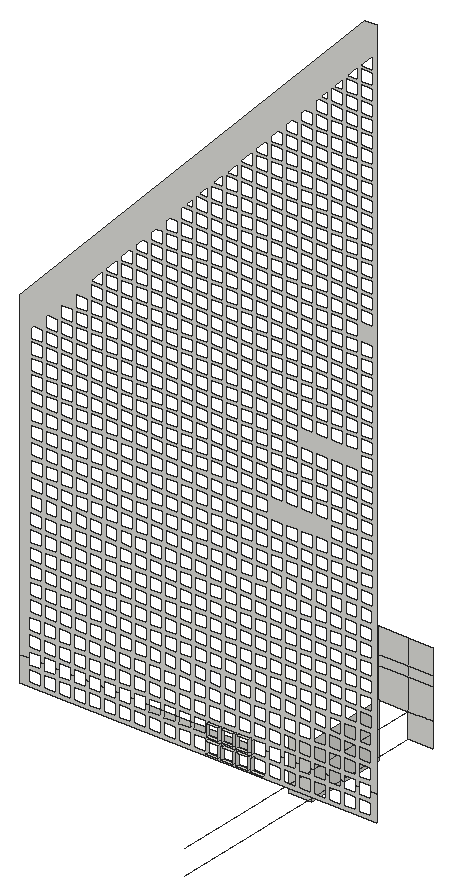
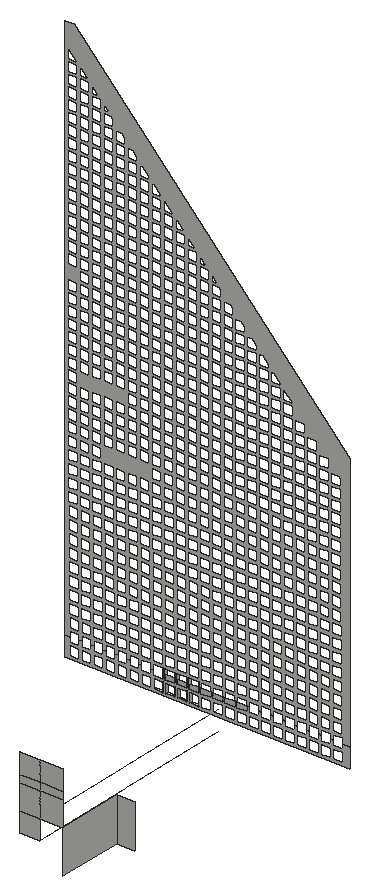
# SketchUp Ruby script. Lengths in inches.
U = 1.inch
M = Sketchup.active_model
def pt(a) = Geom::Point3d.new(a.map { |v| v * U })
def face(e, loops, mat)
  f = e.add_face(loops[0].map { |a| pt(a) })
  loops[1..].each { |l| e.add_face(l.map { |a| pt(a) }).erase! }
  f.material = f.back_material = mat if mat
  f
end
# faces: each face lists its corners as indices into pts; further lists are holes
def faces(e, pts, list, mat = nil) = list.each { |f| face(e, (f[0].is_a?(Array) ? f : [f]).map { |l| l.map { |i| pts[i] } }, mat) }
# xy, xz, yz: faces in a plane at the given z, y or x. An outline is a flat list of corners, or four numbers for a rectangle; further outlines are holes
def ring(l) = l.size == 4 ? [[l[0], l[1]], [l[2], l[1]], [l[2], l[3]], [l[0], l[3]]] : l.each_slice(2).to_a
def flat(e, list, mat, &to3) = list.each { |f| face(e, (f[0].is_a?(Array) ? f : [f]).map { |l| ring(l).map { |u, v| to3.(u, v) } }, mat) }
def xy(e, z, list, mat = nil) = flat(e, list, mat) { |x, y| [x, y, z] }
def xz(e, y, list, mat = nil) = flat(e, list, mat) { |x, z| [x, y, z] }
def yz(e, x, list, mat = nil) = flat(e, list, mat) { |y, z| [x, y, z] }
def lines(e, pts, list) = list.each { |a, b| e.add_line(pt(pts[a]), pt(pts[b])) }
# prism: a flat outline (further loops are holes) pulled along v
def prism(e, loops, v, mat = nil)
  f = face(e, loops, mat); d = Geom::Vector3d.new(v.map { |x| x * U })
  f.pushpull(f.normal.samedirection?(d) ? d.length : -d.length)
end
def box(e, o, s, mat = nil) = prism(e, [[o, [o[0] + s[0], o[1], o[2]], [o[0] + s[0], o[1] + s[1], o[2]], [o[0], o[1] + s[1], o[2]]]], [0, 0, s[2]], mat)
def at(x, y, z, deg = 0) = Geom::Transformation.translation(pt([x, y, z])) * Geom::Transformation.rotation(ORIGIN, Z_AXIS, deg.degrees)
def axes(o, x, y, z) = Geom::Transformation.new([*x, 0, *y, 0, *z, 0, *pt(o).to_a, 1])
def part(name) = M.definitions.add(name)
# library, detail: a bought-in or finely detailed component or shape, given as its bounding box
def library(name, o, s) = part(name).tap { |d| box(d.entities, o, s) }
def detail(e, o, s) = box(e.add_group.entities, o, s)
def put(e, d, t, mat = nil) = e.add_instance(d, t).tap { |i| i.material = mat if mat }
def group(e, t, mat = nil) = e.add_group.tap { |g| g.transformation = t; g.material = mat if mat }.entities
root = M.entities
xy(root,259.68,[[986.41,2332.13,988.72,2332.76],[989.32,2332.13,991.63,2332.76],[992.23,2332.13,994.55,2332.76],[995.15,2332.13,997.46,2332.76]])
xy(root,262,[[986.41,2332.13,988.72,2332.76],[989.32,2332.13,991.63,2332.76],[992.23,2332.13,994.55,2332.76]])
xy(root,262.73,[[986.4375,2332.13,988.75,2332.76],[989.35,2332.13,991.66,2332.76],[992.26,2332.13,994.58,2332.76]])
xy(root,265.04,[[986.4375,2332.13,988.75,2332.76],[989.35,2332.13,991.66,2332.76],[992.26,2332.13,994.58,2332.76]])
xz(root,2332.76,[[[949.71,258.95,949.71,263.89,951.49,263.89,951.49,262.73,953.81,262.73,953.81,263.89,954.41,263.89,954.41,262.73,956.72,262.73,956.72,263.89,957.32,263.89,957.32,262.73,959.63,262.73,959.63,263.89,960.23,263.89,960.23,262.73,962.54,262.73,962.54,263.89,963.14,263.89,963.14,262.73,965.46,262.73,965.46,263.89,966.06,263.89,966.06,262.73,968.37,262.73,968.37,263.89,968.97,263.89,968.97,262.73,971.28,262.73,971.28,263.89,971.88,263.89,971.88,262.73,974.19,262.73,974.19,263.89,974.79,263.89,974.79,262.73,977.1,262.73,977.1,263.89,977.7,263.89,977.7,262.73,980.02,262.73,980.02,263.89,980.62,263.89,980.62,262.73,982.93,262.73,982.93,263.89,983.53,263.89,983.53,262.73,985.84,262.73,985.84,263.89,986.4375,263.89,986.4375,262.73,988.75,262.73,988.75,263.89,989.35,263.89,989.35,262.73,991.66,262.73,991.66,263.89,992.26,263.89,992.26,262.73,994.58,262.73,994.58,263.89,995.18,263.89,995.18,262.73,997.49,262.73,997.49,263.89,998.09,263.89,998.09,262.73,1000.4,262.73,1000.4,263.89,1001,263.89,1001,262.73,1003.3125,262.73,1003.3125,263.89,1003.91,263.89,1003.91,262.73,1006.22,262.73,1006.22,263.89,1006.82,263.89,1006.82,262.73,1009.14,262.73,1009.14,263.89,1009.74,263.89,1009.74,262.73,1012.05,262.73,1012.05,263.89,1012.65,263.89,1012.65,262.73,1014.96,262.73,1014.96,263.89,1015.56,263.89,1015.56,262.73,1017.87,262.73,1017.87,263.89,1019.02,263.89,1019.02,258.95],[1015.53,259.68,1017.84,262],[1012.62,259.68,1014.93,262],[1009.71,259.68,1012.02,262],[1006.79,259.68,1009.11,262],[1003.88,259.68,1006.2,262],[1000.97,259.68,1003.28,262],[998.06,259.68,1000.37,262],[995.15,259.68,997.46,262],[992.23,259.68,994.55,262],[989.32,259.68,991.63,262],[986.41,259.68,988.72,262],[983.5,259.68,985.8125,262],[980.59,259.68,982.9,262],[977.67,259.68,979.99,262],[974.76,259.68,977.07,262],[971.85,259.68,974.16,262],[968.9375,259.68,971.25,262],[966.03,259.68,968.34,262],[963.11,259.68,965.43,262],[960.2,259.68,962.51,262],[957.29,259.68,959.6,262],[954.38,259.68,956.69,262],[951.47,259.68,953.78,262]],[974.79,262.73,977.1,263.89],[977.7,262.73,980.02,263.89],[980.62,262.73,982.93,263.89],[983.53,262.73,985.84,263.89],
  [986.4375,262.73,988.75,263.89],[989.35,262.73,991.66,263.89],[992.26,262.73,994.58,263.89],[[949.71,263.89,949.71,326.5,1016.77,397.75,1019.02,397.75,1019.02,263.89,1017.87,263.89,1017.87,265.04,1015.56,265.04,1015.56,263.89,1014.96,263.89,1014.96,265.04,1012.65,265.04,1012.65,263.89,1012.05,263.89,1012.05,265.04,1009.74,265.04,1009.74,263.89,1009.14,263.89,1009.14,265.04,1006.82,265.04,1006.82,263.89,1006.22,263.89,1006.22,265.04,1003.91,265.04,1003.91,263.89,1003.3125,263.89,1003.3125,265.04,1001,265.04,1001,263.89,1000.4,263.89,1000.4,265.04,998.09,265.04,998.09,263.89,997.49,263.89,997.49,265.04,995.18,265.04,995.18,263.89,994.58,263.89,994.58,265.04,992.26,265.04,992.26,263.89,991.66,263.89,991.66,265.04,989.35,265.04,989.35,263.89,988.75,263.89,988.75,265.04,986.4375,265.04,986.4375,263.89,985.84,263.89,985.84,265.04,983.53,265.04,983.53,263.89,982.93,263.89,982.93,265.04,980.62,265.04,980.62,263.89,980.02,263.89,980.02,265.04,977.7,265.04,977.7,263.89,977.1,263.89,977.1,265.04,974.79,265.04,974.79,263.89,974.19,263.89,974.19,265.04,971.88,265.04,971.88,263.89,971.28,263.89,971.28,265.04,968.97,265.04,968.97,263.89,968.37,263.89,968.37,265.04,966.06,265.04,966.06,263.89,965.46,263.89,965.46,265.04,963.14,265.04,963.14,263.89,962.54,263.89,962.54,265.04,960.23,265.04,960.23,263.89,959.63,263.89,959.63,265.04,957.32,265.04,957.32,263.89,956.72,263.89,956.72,265.04,954.41,265.04,954.41,263.89,953.81,263.89,953.81,265.04,951.49,265.04,951.49,263.89],[1004.32,370.27,1006.66,372.59],[1015.99,386.84,1018.31,389.15],[1015.99,384.09,1018.31,386.4],[1013.08,384.09,1015.4,386.4],[1013.06,381.34,1015.37,383.65],[1015.99,381.34,1018.31,383.65],[1015.99,378.59,1018.31,380.9],[1013.06,378.59,1015.37,380.9],[1010.15,375.84,1012.46,378.15],[1013.08,375.84,1015.4,378.15],[1015.99,375.84,1018.31,378.15],[1015.99,373.09,1018.31,375.4],[1013.06,373.09,1015.37,375.4],[1010.17,373.09,1012.48,375.4],[1007.23,373.09,1009.55,375.4],[1013.06,370.27,1015.37,372.59],[1015.99,370.27,1018.31,372.59],[1007.26,370.27,1009.57,372.59],[1001.43,370.27,1003.75,372.59],[998.52,367.46,1000.83,369.77],[1001.43,367.46,1003.75,369.77],[1004.35,367.46,1006.66,369.77],[1007.26,367.46,1009.57,369.77],[1010.17,367.46,1012.48,369.77],[1013.08,367.46,1015.4,369.77],[1015.99,367.46,1018.31,369.77],[1015.99,364.65,1018.31,366.96],[1013.08,364.65,1015.4,366.96],[1010.17,364.65,1012.48,366.96],[1007.26,364.65,1009.57,366.96],[1004.35,364.65,1006.66,366.96],[1001.43,364.65,1003.75,366.96],[998.52,364.65,1000.83,366.96],[995.61,364.65,997.92,366.96],[992.7,361.84,995.01,364.15],[995.61,361.84,997.92,364.15],[998.52,361.84,1000.83,364.15],[1001.43,361.84,1003.75,364.15],[1004.35,361.84,1006.66,364.15],[1007.26,361.84,1009.57,364.15],[1010.17,361.84,1012.48,364.15],[1013.08,361.84,1015.4,364.15],[1015.99,361.84,1018.31,364.15],[1015.99,359.02,1018.31,361.34],[1013.08,359.02,1015.4,361.34],[1010.17,359.02,1012.48,361.34],[1007.26,359.02,1009.57,361.34],[1004.35,359.02,1006.66,361.34],[1001.43,359.02,1003.75,361.34],[998.52,359.02,1000.83,361.34],[995.61,359.02,997.92,361.34],[992.7,359.02,995.01,361.34],[989.79,359.02,992.1,361.34],[986.875,356.21,989.1875,358.52],[989.79,356.21,992.1,358.52],[992.7,356.21,995.01,358.52],[995.61,356.21,997.92,358.52],[998.52,356.21,1000.83,358.52],[1001.43,356.21,1003.75,358.52],[1004.35,356.21,1006.66,358.52],[1007.26,356.21,1009.57,358.52],[1010.17,356.21,1012.48,358.52],[1013.08,356.21,1015.4,358.52],[1015.99,356.21,1018.31,358.52],[983.96,350.59,986.27,352.9],[986.875,353.4,989.1875,355.71],[986.875,350.59,989.1875,352.9],[989.79,350.59,992.1,352.9],[989.79,353.4,992.1,355.71],[992.7,353.4,995.01,355.71],[992.7,350.59,995.01,352.9],[995.61,353.4,997.92,355.71],[995.61,350.59,997.92,352.9],[998.52,353.4,1000.83,355.71],[998.52,350.59,1000.83,352.9],[1001.43,353.4,1003.75,355.71],[1001.43,350.59,1003.75,352.9],[1004.35,353.4,1006.66,355.71],[1004.35,350.59,1006.66,352.9],[1007.26,350.59,1009.57,352.9],[1007.26,353.4,1009.57,355.71],[1010.17,353.4,1012.48,355.71],[1013.08,353.4,1015.4,355.71],[1015.99,353.4,1018.31,355.71],[1015.99,350.59,1018.31,352.9],[1013.08,350.59,1015.4,352.9],[1010.17,350.59,1012.48,352.9],[1015.99,347.77,1018.31,350.09],[1013.08,347.77,1015.4,350.09],[1010.17,347.77,1012.48,350.09],[1007.26,347.77,1009.57,350.09],[1004.35,347.77,1006.66,350.09],[1001.43,347.77,1003.75,350.09],[998.52,347.77,1000.83,350.09],[995.61,347.77,997.92,350.09],[992.7,347.77,995.01,350.09],[989.79,347.77,992.1,350.09],[986.875,347.77,989.1875,350.09],[983.96,347.77,986.27,350.09],[981.05,347.77,983.36,350.09],[978.14,344.96,980.45,347.27],[981.05,344.96,983.36,347.27],[983.96,344.96,986.27,347.27],[986.875,344.96,989.1875,347.27],[989.79,344.96,992.1,347.27],[992.7,344.96,995.01,347.27],[995.61,344.96,997.92,347.27],[998.52,344.96,1000.83,347.27],[1001.43,344.96,1003.75,347.27],[1004.35,344.96,1006.66,347.27],[1007.26,344.96,1009.57,347.27],[1010.17,344.96,1012.48,347.27],[1013.08,344.96,1015.4,347.27],[1015.99,344.96,1018.31,347.27],[969.4,336.52,971.71,338.84],[972.3125,336.52,974.625,338.84],[975.23,336.52,977.54,338.84],[978.14,336.52,980.45,338.84],[981.05,336.52,983.36,338.84],[983.96,336.52,986.27,338.84],[986.875,336.52,989.1875,338.84],[989.79,336.52,992.1,338.84],[992.7,336.52,995.01,338.84],[995.61,336.52,997.92,338.84],[995.61,339.34,997.92,341.65],[992.7,339.34,995.01,341.65],[989.79,339.34,992.1,341.65],[986.875,339.34,989.1875,341.65],[983.96,339.34,986.27,341.65],[981.05,339.34,983.36,341.65],[978.14,339.34,980.45,341.65],[975.23,339.34,977.54,341.65],[972.3125,339.34,974.625,341.65],[975.23,342.15,977.54,344.46],[978.14,342.15,980.45,344.46],[981.05,342.15,983.36,344.46],[983.96,342.15,986.27,344.46],[986.875,342.15,989.1875,344.46],[989.79,342.15,992.1,344.46],[992.7,342.15,995.01,344.46],[995.61,342.15,997.92,344.46],[998.52,342.15,1000.83,344.46],[998.52,339.34,1000.83,341.65],[998.52,336.52,1000.83,338.84],[1001.43,336.52,1003.75,338.84],[1001.43,339.34,1003.75,341.65],[1001.43,342.15,1003.75,344.46],[1004.35,342.15,1006.66,344.46],[1004.35,339.34,1006.66,341.65],[1004.35,336.52,1006.66,338.84],[1007.26,336.52,1009.57,338.84],[1007.26,339.34,1009.57,341.65],[1007.26,342.15,1009.57,344.46],[1010.17,342.15,1012.48,344.46],[1010.17,339.34,1012.48,341.65],[1010.17,336.52,1012.48,338.84],[1013.08,336.52,1015.4,338.84],[1013.08,339.34,1015.4,341.65],[1013.08,342.15,1015.4,344.46],[1015.99,339.34,1018.31,341.65],[1015.99,336.52,1018.31,338.84],[1015.99,333.71,1018.31,336.02],[1013.08,333.71,1015.4,336.02],[1010.17,333.71,1012.48,336.02],[1007.26,333.71,1009.57,336.02],[1004.35,333.71,1006.66,336.02],[1001.43,333.71,1003.75,336.02],[998.52,333.71,1000.83,336.02],[995.61,333.71,997.92,336.02],[992.7,333.71,995.01,336.02],[989.79,333.71,992.1,336.02],[986.875,333.71,989.1875,336.02],[983.96,333.71,986.27,336.02],[981.05,333.71,983.36,336.02],[978.14,333.71,980.45,336.02],[975.23,333.71,977.54,336.02],[972.3125,333.71,974.625,336.02],[969.4,333.71,971.71,336.02],[966.49,333.71,968.8,336.02],[963.58,330.9,965.89,333.21],[966.49,330.9,968.8,333.21],[969.4,330.9,971.71,333.21],[972.3125,330.9,974.625,333.21],[975.23,330.9,977.54,333.21],[978.14,330.9,980.45,333.21],[981.05,330.9,983.36,333.21],[983.96,330.9,986.27,333.21],[986.875,330.9,989.1875,333.21],[989.79,330.9,992.1,333.21],[992.7,330.9,995.01,333.21],[995.61,330.9,997.92,333.21],[998.52,330.9,1000.83,333.21],[1001.43,330.9,1003.75,333.21],[1004.35,330.9,1006.66,333.21],[1007.26,330.9,1009.57,333.21],[1010.17,330.9,1012.48,333.21],[1013.08,330.9,1015.4,333.21],[1015.99,330.9,1018.31,333.21],[1015.99,328.09,1018.31,330.4],[1013.08,328.09,1015.4,330.4],[1010.17,328.09,1012.48,330.4],[1007.26,328.09,1009.57,330.4],[1004.35,328.09,1006.66,330.4],[1001.43,328.09,1003.75,330.4],[998.52,328.09,1000.83,330.4],[995.61,328.09,997.92,330.4],[992.7,328.09,995.01,330.4],[989.79,328.09,992.1,330.4],[986.875,328.09,989.1875,330.4],[983.96,328.09,986.27,330.4],[981.05,328.09,983.36,330.4],[978.14,328.09,980.45,330.4],[975.23,328.09,977.54,330.4],[972.3125,328.09,974.625,330.4],[969.4,328.09,971.71,330.4],[966.49,328.09,968.8,330.4],[963.58,328.09,965.89,330.4],[960.67,328.09,962.98,330.4],[957.75,325.27,960.07,327.59],[960.67,325.27,962.98,327.59],[963.58,325.27,965.89,327.59],[966.49,325.27,968.8,327.59],[969.4,325.27,971.71,327.59],[972.3125,325.27,974.625,327.59],[975.23,325.27,977.54,327.59],[978.14,325.27,980.45,327.59],[981.05,325.27,983.36,327.59],[983.96,325.27,986.27,327.59],[986.875,325.27,989.1875,327.59],[989.79,325.27,992.1,327.59],[992.7,325.27,995.01,327.59],[995.61,325.27,997.92,327.59],[998.52,325.27,1000.83,327.59],[1001.43,325.27,1003.75,327.59],[1004.35,325.27,1006.66,327.59],[1007.26,325.27,1009.57,327.59],[1010.17,325.27,1012.48,327.59],[1013.08,325.27,1015.4,327.59],[1015.99,325.27,1018.31,327.59],[1015.99,322.46,1018.31,324.77],[1013.08,322.46,1015.4,324.77],[1010.17,322.46,1012.48,324.77],[1007.26,322.46,1009.57,324.77],[1004.35,322.46,1006.66,324.77],[1001.43,322.46,1003.75,324.77],[998.52,322.46,1000.83,324.77],[995.61,322.46,997.92,324.77],[992.7,322.46,995.01,324.77],[989.79,322.46,992.1,324.77],[986.875,322.46,989.1875,324.77],[983.96,322.46,986.27,324.77],[981.05,322.46,983.36,324.77],[978.14,322.46,980.45,324.77],[978.14,319.65,980.45,321.96],[981.05,319.65,983.36,321.96],[983.96,319.65,986.27,321.96],[986.875,319.65,989.1875,321.96],[989.79,319.65,992.1,321.96],[992.7,319.65,995.01,321.96],[995.61,319.65,997.92,321.96],[998.52,319.65,1000.83,321.96],[1001.43,319.65,1003.75,321.96],[1015.99,319.65,1018.31,321.96],[1015.99,316.84,1018.31,319.15],[1013.08,316.84,1015.4,319.15],[1010.17,316.84,1012.48,319.15],[1007.26,316.84,1009.57,319.15],[1004.35,316.84,1006.66,319.15],[1001.43,316.84,1003.75,319.15],[998.52,316.84,1000.83,319.15],[995.61,316.84,997.92,319.15],[992.7,316.84,995.01,319.15],[989.79,316.84,992.1,319.15],[986.875,316.84,989.1875,319.15],[983.96,316.84,986.27,319.15],[981.05,316.84,983.36,319.15],[978.14,316.84,980.45,319.15],[978.14,314.02,980.45,316.34],[981.05,314.02,983.36,316.34],[983.96,314.02,986.27,316.34],[986.875,314.02,989.1875,316.34],[989.79,314.02,992.1,316.34],[992.7,314.02,995.01,316.34],[995.61,314.02,997.92,316.34],[998.52,314.02,1000.83,316.34],[1001.43,314.02,1003.75,316.34],[1004.35,314.02,1006.66,316.34],[1007.26,314.02,1009.57,316.34],[1010.17,314.02,1012.48,316.34],[1013.08,314.02,1015.4,316.34],[1015.99,314.02,1018.31,316.34],[957.75,322.46,960.07,324.77],[960.67,322.46,962.98,324.77],[963.58,322.46,965.89,324.77],[966.49,322.46,968.8,324.77],[969.4,322.46,971.71,324.77],[972.3125,322.46,974.625,324.77],[975.23,322.46,977.54,324.77],[975.23,319.65,977.54,321.96],[975.23,316.84,977.54,319.15],[975.23,314.02,977.54,316.34],[972.3125,314.02,974.625,316.34],[972.3125,316.84,974.625,319.15],[972.3125,319.65,974.625,321.96],[969.4,319.65,971.71,321.96],[966.49,319.65,968.8,321.96],[963.58,319.65,965.89,321.96],[960.67,319.65,962.98,321.96],[957.75,319.65,960.07,321.96],[954.84,319.65,957.15,321.96],[951.93,316.84,954.24,319.15],[954.84,316.84,957.15,319.15],[957.75,316.84,960.07,319.15],[960.67,316.84,962.98,319.15],[963.58,316.84,965.89,319.15],[966.49,316.84,968.8,319.15],[969.4,316.84,971.71,319.15],[969.4,314.02,971.71,316.34],[966.49,314.02,968.8,316.34],[963.58,314.02,965.89,316.34],[960.67,314.02,962.98,316.34],[957.75,314.02,960.07,316.34],[954.84,314.02,957.15,316.34],[951.93,314.02,954.24,316.34],[951.93,311.21,954.24,313.52],[954.84,311.21,957.15,313.52],[957.75,311.21,960.07,313.52],[960.67,311.21,962.98,313.52],[963.58,311.21,965.89,313.52],[966.49,311.21,968.8,313.52],[969.4,311.21,971.71,313.52],[972.3125,311.21,974.625,313.52],[975.23,311.21,977.54,313.52],[978.14,311.21,980.45,313.52],[981.05,311.21,983.36,313.52],[983.96,311.21,986.27,313.52],[986.875,311.21,989.1875,313.52],[989.79,311.21,992.1,313.52],[992.7,311.21,995.01,313.52],[995.61,311.21,997.92,313.52],[998.52,311.21,1000.83,313.52],[1001.43,311.21,1003.75,313.52],[1004.35,311.21,1006.66,313.52],[1007.26,311.21,1009.57,313.52],[1010.17,311.21,1012.48,313.52],[1013.08,311.21,1015.4,313.52],[1015.99,311.21,1018.31,313.52],[951.93,308.4,954.24,310.71],[954.84,308.4,957.15,310.71],[957.75,308.4,960.07,310.71],[960.67,308.4,962.98,310.71],[963.58,308.4,965.89,310.71],[966.49,308.4,968.8,310.71],[969.4,308.4,971.71,310.71],[972.3125,308.4,974.625,310.71],[975.23,308.4,977.54,310.71],[978.14,308.4,980.45,310.71],[981.05,308.4,983.36,310.71],[983.96,308.4,986.27,310.71],[986.875,308.4,989.1875,310.71],[989.79,308.4,992.1,310.71],[992.7,308.4,995.01,310.71],[995.61,308.4,997.92,310.71],[998.52,308.4,1000.83,310.71],[1001.43,308.4,1003.75,310.71],[1004.35,308.4,1006.66,310.71],[1007.26,308.4,1009.57,310.71],[1010.17,308.4,1012.48,310.71],[1013.08,308.4,1015.4,310.71],[1015.99,308.4,1018.31,310.71],[1015.97,305.35,1018.28,307.67],[1013.05,305.35,1015.37,307.67],[1010.14,305.35,1012.45,307.67],[995.58,305.35,997.89,307.67],[992.67,305.35,994.98,307.67],[989.76,305.35,992.07,307.67],[986.85,305.35,989.16,307.67],[983.93,305.35,986.25,307.67],[981.02,305.35,983.33,307.67],[978.11,305.35,980.42,307.67],[975.2,305.35,977.51,307.67],[972.29,305.35,974.6,307.67],[969.375,305.35,971.6875,307.67],[966.46,305.35,968.77,307.67],[963.55,305.35,965.86,307.67],[960.64,305.35,962.95,307.67],[957.72,305.35,960.04,307.67],[954.8125,305.35,957.125,307.67],[951.9,305.35,954.21,307.67],[951.87,302.31,954.18,304.62],[954.78,302.31,957.1,304.62],[957.7,302.31,960.01,304.62],[960.61,302.31,962.92,304.62],[963.52,302.31,965.83,304.62],[966.43,302.31,968.74,304.62],[969.34,302.31,971.66,304.62],[972.26,302.31,974.57,304.62],[975.17,302.31,977.48,304.62],[978.08,302.31,980.39,304.62],[980.99,302.31,983.3,304.62],[983.9,302.31,986.22,304.62],[986.82,302.31,989.13,304.62],[989.73,302.31,992.04,304.62],[992.64,302.31,994.95,304.62],[995.55,302.31,997.86,304.62],[998.46,302.31,1000.78,304.62],[1001.375,302.31,1003.6875,304.62],[1004.29,302.31,1006.6,304.62],[1007.2,302.31,1009.51,304.62],[1010.11,302.31,1012.43,304.62],[1013.02,302.31,1015.34,304.62],[1015.9375,302.31,1018.25,304.62],[1015.91,299.27,1018.22,301.58],[1013,299.27,1015.31,301.58],[1010.08,299.27,1012.4,301.58],[1007.17,299.27,1009.48,301.58],[1004.26,299.27,1006.57,301.58],[1001.35,299.27,1003.66,301.58],[998.44,299.27,1000.75,301.58],[995.52,299.27,997.84,301.58],[992.61,299.27,994.92,301.58],[989.7,299.27,992.01,301.58],[986.79,299.27,989.1,301.58],[983.875,299.27,986.1875,301.58],[980.96,299.27,983.28,301.58],[978.05,299.27,980.36,301.58],[975.14,299.27,977.45,301.58],[972.23,299.27,974.54,301.58],[969.32,299.27,971.63,301.58],[966.4,299.27,968.72,301.58],[963.49,299.27,965.8,301.58],[960.58,299.27,962.89,301.58],[957.67,299.27,959.98,301.58],[954.75,299.27,957.07,301.58],[951.84,299.27,954.16,301.58],[951.8125,296.22,954.125,298.53],[954.73,296.22,957.04,298.53],[957.64,296.22,959.95,298.53],[960.55,296.22,962.86,298.53],[963.46,296.22,965.77,298.53],[966.375,296.22,968.6875,298.53],[969.29,296.22,971.6,298.53],[972.2,296.22,974.51,298.53],[975.11,296.22,977.42,298.53],[978.02,296.22,980.33,298.53],[980.93,296.22,983.25,298.53],[983.85,296.22,986.16,298.53],[986.76,296.22,989.07,298.53],[989.67,296.22,991.98,298.53],[992.58,296.22,994.89,298.53],[995.49,296.22,997.81,298.53],[998.41,296.22,1000.72,298.53],[1001.32,296.22,1003.63,298.53],[1004.23,296.22,1006.54,298.53],[1007.14,296.22,1009.46,298.53],[1010.05,296.22,1012.37,298.53],[1012.97,296.22,1015.28,298.53],[1015.88,296.22,1018.19,298.53],[951.78,293.18,954.1,295.49],[954.7,293.18,957.01,295.49],[957.61,293.18,959.92,295.49],[960.52,293.18,962.83,295.49],[963.43,293.18,965.75,295.49],[966.35,293.18,968.66,295.49],[969.26,293.18,971.57,295.49],[972.17,293.18,974.48,295.49],[975.08,293.18,977.39,295.49],[977.99,293.18,980.31,295.49],[980.91,293.18,983.22,295.49],[983.82,293.18,986.13,295.49],[986.73,293.18,989.04,295.49],[989.64,293.18,991.95,295.49],[992.55,293.18,994.87,295.49],[995.47,293.18,997.78,295.49],[998.38,293.18,1000.69,295.49],[1001.29,293.18,1003.6,295.49],[1004.2,293.18,1006.51,295.49],[1007.11,293.18,1009.43,295.49],[1010.03,293.18,1012.34,295.49],[1012.9375,293.18,1015.25,295.49],[1015.85,293.18,1018.16,295.49],[963.4,290.13,965.72,292.44],[966.32,290.13,968.63,292.44],[969.23,290.13,971.54,292.44],[972.14,290.13,974.45,292.44],[975.05,290.13,977.36,292.44],[977.96,290.13,980.28,292.44],[980.875,290.13,983.1875,292.44],[983.79,290.13,986.1,292.44],[986.7,290.13,989.01,292.44],[989.61,290.13,991.92,292.44],[992.52,290.13,994.84,292.44],[995.4375,290.13,997.75,292.44],[998.35,290.13,1000.66,292.44],[1001.26,290.13,1003.57,292.44],[1004.17,290.13,1006.49,292.44],[1007.08,290.13,1009.4,292.44],[1010,290.13,1012.31,292.44],[1012.91,290.13,1015.22,292.44],[1015.82,290.13,1018.13,292.44],[1015.79,287.09,1018.1,289.4],[1012.88,287.09,1015.19,289.4],[1009.97,287.09,1012.28,289.4],[1007.06,287.09,1009.37,289.4],[1004.14,287.09,1006.46,289.4],[1001.23,287.09,1003.54,289.4],[998.32,287.09,1000.63,289.4],[995.41,287.09,997.72,289.4],[992.5,287.09,994.81,289.4],[989.58,287.09,991.9,289.4],[986.67,287.09,988.98,289.4],[983.76,287.09,986.07,289.4],[980.85,287.09,983.16,289.4],[977.94,287.09,980.25,289.4],[975.02,287.09,977.34,289.4],[972.11,287.09,974.42,289.4],[969.2,287.09,971.51,289.4],[966.29,287.09,968.6,289.4],[963.375,287.09,965.6875,289.4],[963.35,284.04,965.66,286.35],[966.26,284.04,968.57,286.35],[969.17,284.04,971.48,286.35],[972.08,284.04,974.39,286.35],[974.99,284.04,977.31,286.35],[977.91,284.04,980.22,286.35],[980.82,284.04,983.13,286.35],[983.73,284.04,986.04,286.35],[986.64,284.04,988.95,286.35],[989.55,284.04,991.87,286.35],[992.47,284.04,994.78,286.35],[995.38,284.04,997.69,286.35],[998.29,284.04,1000.6,286.35],[1001.2,284.04,1003.52,286.35],[1004.11,284.04,1006.43,286.35],[1007.03,284.04,1009.34,286.35],[1009.9375,284.04,1012.25,286.35],[1012.85,284.04,1015.16,286.35],[1015.76,284.04,1018.08,286.35],[1015.73,281,1018.05,283.31],[1012.82,281,1015.13,283.31],[1009.91,281,1012.22,283.31],[1007,281,1009.31,283.31],[1004.09,281,1006.4,283.31],[1001.17,281,1003.49,283.31],[998.26,281,1000.57,283.31],[995.35,281,997.66,283.31],[992.4375,281,994.75,283.31],[989.53,281,991.84,283.31],[986.61,281,988.93,283.31],[983.7,281,986.01,283.31],[980.79,281,983.1,283.31],[977.88,281,980.19,283.31],[974.97,281,977.28,283.31],[972.05,281,974.37,283.31],[969.14,281,971.45,283.31],[966.23,281,968.54,283.31],[966.2,277.95,968.51,280.26],[969.11,277.95,971.42,280.26],[972.02,277.95,974.34,280.26],[974.9375,277.95,977.25,280.26],[977.85,277.95,980.16,280.26],[980.76,277.95,983.07,280.26],[983.67,277.95,985.98,280.26],[986.58,277.95,988.9,280.26],[989.5,277.95,991.81,280.26],[992.41,277.95,994.72,280.26],[995.32,277.95,997.63,280.26],[998.23,277.95,1000.55,280.26],[1001.14,277.95,1003.46,280.26],[1004.06,277.95,1006.37,280.26],[1006.97,277.95,1009.28,280.26],[1009.88,277.95,1012.19,280.26],[1012.79,277.95,1015.11,280.26],[1015.7,277.95,1018.02,280.26],[1015.68,274.91,1017.99,277.22],[1012.76,274.91,1015.08,277.22],[1009.85,274.91,1012.16,277.22],[1006.94,274.91,1009.25,277.22],[1004.03,274.91,1006.34,277.22],[1001.12,274.91,1003.43,277.22],[998.2,274.91,1000.52,277.22],[995.29,274.91,997.6,277.22],[992.38,274.91,994.69,277.22],[989.47,274.91,991.78,277.22],[986.56,274.91,988.87,277.22],[983.64,274.91,985.96,277.22],[980.73,274.91,983.04,277.22],[977.82,274.91,980.13,277.22],[974.91,274.91,977.22,277.22],[972,274.91,974.31,277.22],[969.08,274.91,971.4,277.22],[966.17,274.91,968.48,277.22],[963.32,281,965.63,283.31],[963.29,277.95,965.6,280.26],[963.26,274.91,965.57,277.22],[960.35,274.91,962.66,277.22],[960.375,277.95,962.6875,280.26],[960.41,281,962.72,283.31],[960.43,284.04,962.75,286.35],[960.46,287.09,962.78,289.4],[960.49,290.13,962.8,292.44],[957.58,290.13,959.89,292.44],[957.55,287.09,959.86,289.4],[957.52,284.04,959.83,286.35],[957.49,281,959.81,283.31],[954.55,277.95,956.86,280.26],[957.46,277.95,959.78,280.26],[957.44,274.91,959.75,277.22],[954.52,274.91,956.84,277.22],[954.58,281,956.89,283.31],[954.61,284.04,956.92,286.35],[954.64,287.09,956.95,289.4],[954.67,290.13,956.98,292.44],[951.76,290.13,954.07,292.44],[951.73,287.09,954.04,289.4],[951.7,284.04,954.01,286.35],[951.67,281,953.98,283.31],[951.64,277.95,953.95,280.26],[951.61,274.91,953.92,277.22],[951.58,271.86,953.89,274.17],[954.49,271.86,956.81,274.17],[957.41,271.86,959.72,274.17],[960.32,271.86,962.63,274.17],[963.23,271.86,965.54,274.17],[966.14,271.86,968.45,274.17],[969.05,271.86,971.37,274.17],[971.97,271.86,974.28,274.17],[974.88,271.86,977.19,274.17],[977.79,271.86,980.1,274.17],[980.7,271.86,983.01,274.17],[983.61,271.86,985.93,274.17],[986.53,271.86,988.84,274.17],[989.4375,271.86,991.75,274.17],[992.35,271.86,994.66,274.17],[995.26,271.86,997.57,274.17],[998.17,271.86,1000.49,274.17],[1001.09,271.86,1003.4,274.17],[1004,271.86,1006.3125,274.17],[1006.91,271.86,1009.22,274.17],[1009.82,271.86,1012.14,274.17],[1012.73,271.86,1015.05,274.17],[1015.65,271.86,1017.96,274.17],[1015.62,268.82,1017.93,271.13],[1012.71,268.82,1015.02,271.13],[1009.79,268.82,1012.11,271.13],[1006.88,268.82,1009.19,271.13],[1003.97,268.82,1006.28,271.13],[1001.06,268.82,1003.37,271.13],[998.15,268.82,1000.46,271.13],[995.23,268.82,997.55,271.13],[992.32,268.82,994.63,271.13],[989.41,268.82,991.72,271.13],[986.5,268.82,988.81,271.13],[983.59,268.82,985.9,271.13],[980.67,268.82,982.99,271.13],[977.76,268.82,980.07,271.13],[974.85,268.82,977.16,271.13],[971.9375,268.82,974.25,271.13],[969.03,268.82,971.34,271.13],[966.11,268.82,968.43,271.13],[963.2,268.82,965.51,271.13],[960.29,268.82,962.6,271.13],[957.38,268.82,959.69,271.13],[954.46,268.82,956.78,271.13],[951.55,268.82,953.87,271.13],[951.52,265.77,953.84,268.09],[954.4375,265.77,956.75,268.09],[957.35,265.77,959.66,268.09],[960.26,265.77,962.57,268.09],[963.17,265.77,965.48,268.09],[966.08,265.77,968.4,268.09],[969,265.77,971.31,268.09],[971.91,265.77,974.22,268.09],[974.82,265.77,977.13,268.09],[977.73,265.77,980.04,268.09],[980.64,265.77,982.96,268.09],[983.56,265.77,985.87,268.09],[986.47,265.77,988.78,268.09],[989.38,265.77,991.69,268.09],[992.29,265.77,994.6,268.09],[995.2,265.77,997.52,268.09],[998.12,265.77,1000.43,268.09],[1001.03,265.77,1003.34,268.09],[1003.94,265.77,1006.25,268.09],[1006.85,265.77,1009.17,268.09],[1009.76,265.77,1012.08,268.09],[1012.68,265.77,1014.99,268.09],[1015.59,265.77,1017.9,268.09],[1010.17,381.34,1012.48,381.34,1012.48,383.65,1010.28,383.65,1010.17,383.53],[1010.17,378.59,1012.48,378.59,1012.48,380.9,1010.28,380.9,1010.17,380.78],[1007.26,375.84,1009.57,375.84,1009.57,378.15,1007.37,378.15,1007.26,378.03],[1010.17,370.27,1012.48,370.27,1012.48,372.59,1010.28,372.59,1010.17,372.47],[1004.35,373.09,1006.66,373.09,1006.66,375.4,1004.46,375.4,1004.35,375.28],[983.96,353.4,986.27,353.4,986.27,355.71,984.09,355.71,983.96,355.57],[954.84,322.46,957.15,322.46,957.15,324.77,955.1,324.77,954.84,324.5],[981.05,350.59,983.36,350.59,983.36,352.9,981.46,352.9,981.05,352.46],[1007.26,378.59,1009.57,378.59,1009.57,380.9,1007.7,380.9,1007.26,380.43],[951.93,319.65,954.24,319.65,954.24,321.96,952.46,321.96,951.93,321.39],[978.14,347.77,980.45,347.77,980.45,350.09,978.82,350.09,978.14,349.36],[1004.35,375.84,1006.66,375.84,1006.66,378.15,1005.125,378.15,1004.35,377.32],[975.23,344.96,977.54,344.96,977.54,347.27,976.1875,347.27,975.23,346.25],[1001.43,373.09,1003.75,373.09,1003.75,375.4,1002.55,375.4,1001.43,374.21],[972.3125,342.15,974.625,342.15,974.625,344.46,973.55,344.46,972.3125,343.14],[998.52,370.27,1000.83,370.27,1000.83,372.59,999.91,372.59,998.52,371.11],[969.4,339.34,971.71,339.34,971.71,341.65,970.91,341.65,969.4,340.04],[995.61,367.46,997.92,367.46,997.92,369.77,997.27,369.77,995.61,368],[966.49,336.52,968.8,336.52,968.8,338.84,968.28,338.84,966.49,336.93],[992.7,364.65,995.01,364.65,995.01,366.96,994.64,366.96,992.7,364.89],[1015.99,389.59,1018.31,389.59,1018.31,391.9,1018.01,391.9,1015.99,389.75],[963.58,333.71,965.89,333.71,965.89,336.02,965.64,336.02,963.58,333.82],[989.84,361.84,992.1,361.84,992.1,364.15,992,364.15],[1013.27,386.84,1015.4,386.84,1015.4,389.11],[987.2,359.02,989.1875,359.02,989.1875,361.14],[1010.69,384.09,1012.48,384.09,1012.48,386],[984.5625,356.21,986.27,356.21,986.27,358.04],[1008.11,381.34,1009.57,381.34,1009.57,382.89],[981.93,353.4,983.36,353.4,983.36,354.93]]])
xz(root,2357.31,[[982.37,240.47,986.75,251.0625]])
xz(root,2373.56,[[992.47,246.25,997.28,251.0625],[986.75,251.0625,992.47,257.0625],[992.47,251.0625,997.28,257.0625],[986.75,257.0625,992.47,258.95],[992.47,257.0625,997.28,258.95],
  [986.75,258.95,992.47,263.89],[992.47,258.95,997.28,263.89]])
yz(root,986.4375,[[2332.13,262.73,2332.76,265.04]])
yz(root,986.75,[[2357.31,240.47,2373.56,251.0625]])
yz(root,988.72,[[2332.13,259.68,2332.76,262]])
yz(root,988.75,[[2332.13,262.73,2332.76,265.04]])
yz(root,989.32,[[2332.13,259.68,2332.76,262]])
yz(root,989.35,[[2332.13,262.73,2332.76,265.04]])
yz(root,991.63,[[2332.13,259.68,2332.76,262]])
yz(root,991.66,[[2332.13,262.73,2332.76,265.04]])
yz(root,992.23,[[2332.13,259.68,2332.76,262]])
yz(root,992.26,[[2332.13,262.73,2332.76,265.04]])
yz(root,994.55,[[2332.13,259.68,2332.76,262]])
yz(root,994.58,[[2332.13,262.73,2332.76,265.04]])
yz(root,995.15,[[2332.13,259.68,2332.76,262]])
yz(root,995.18,[[2332.13,262.73,2332.76,265.04]])
p = [[992.47,2373.56,246.25],[992.47,2319.18,246.25],[992.47,2373.56,251.0625],[992.47,2319.18,251.0625]]
lines(root,p,[[0,1],[2,3]])
